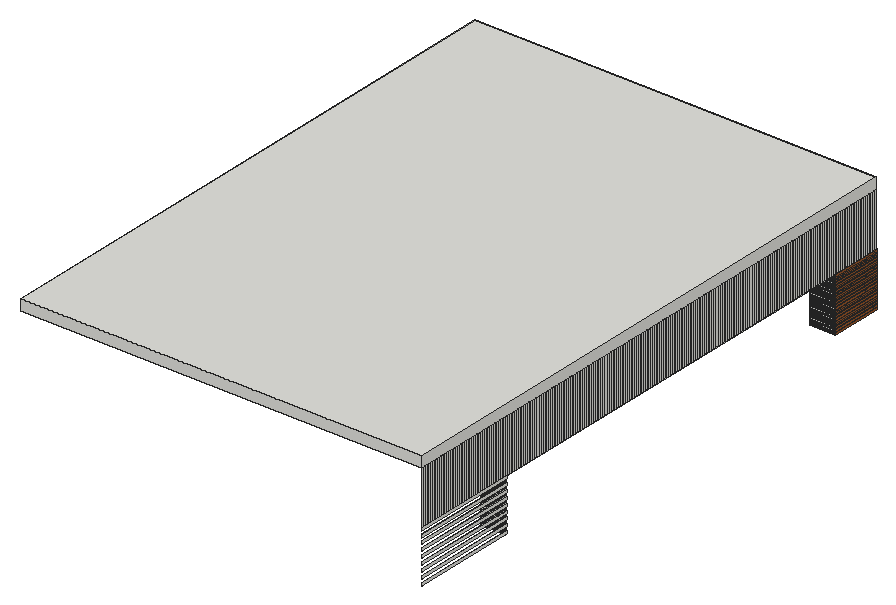
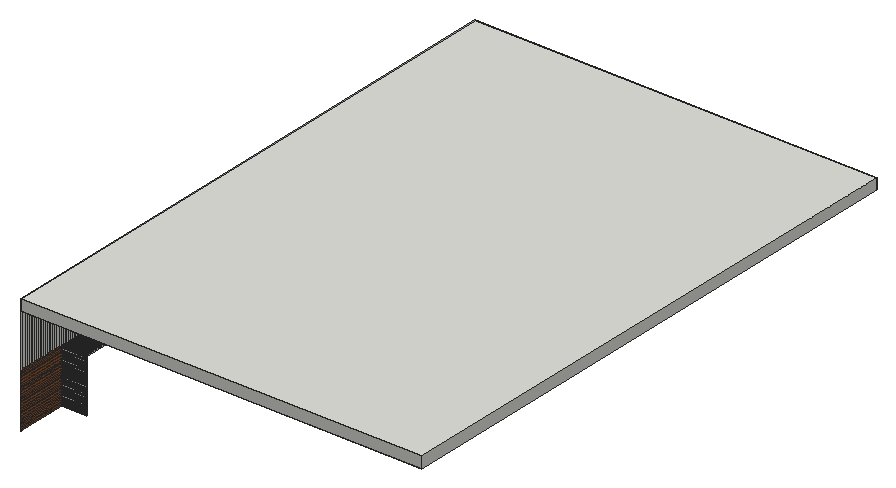
# SketchUp Ruby script. Lengths in inches.
U = 1.inch
M = Sketchup.active_model
def pt(a) = Geom::Point3d.new(a.map { |v| v * U })
def face(e, loops, mat)
  f = e.add_face(loops[0].map { |a| pt(a) })
  loops[1..].each { |l| e.add_face(l.map { |a| pt(a) }).erase! }
  f.material = f.back_material = mat if mat
  f
end
# faces: each face lists its corners as indices into pts; further lists are holes
def faces(e, pts, list, mat = nil) = list.each { |f| face(e, (f[0].is_a?(Array) ? f : [f]).map { |l| l.map { |i| pts[i] } }, mat) }
# xy, xz, yz: faces in a plane at the given z, y or x. An outline is a flat list of corners, or four numbers for a rectangle; further outlines are holes
def ring(l) = l.size == 4 ? [[l[0], l[1]], [l[2], l[1]], [l[2], l[3]], [l[0], l[3]]] : l.each_slice(2).to_a
def flat(e, list, mat, &to3) = list.each { |f| face(e, (f[0].is_a?(Array) ? f : [f]).map { |l| ring(l).map { |u, v| to3.(u, v) } }, mat) }
def xy(e, z, list, mat = nil) = flat(e, list, mat) { |x, y| [x, y, z] }
def xz(e, y, list, mat = nil) = flat(e, list, mat) { |x, z| [x, y, z] }
def yz(e, x, list, mat = nil) = flat(e, list, mat) { |y, z| [x, y, z] }
def lines(e, pts, list) = list.each { |a, b| e.add_line(pt(pts[a]), pt(pts[b])) }
# prism: a flat outline (further loops are holes) pulled along v
def prism(e, loops, v, mat = nil)
  f = face(e, loops, mat); d = Geom::Vector3d.new(v.map { |x| x * U })
  f.pushpull(f.normal.samedirection?(d) ? d.length : -d.length)
end
def box(e, o, s, mat = nil) = prism(e, [[o, [o[0] + s[0], o[1], o[2]], [o[0] + s[0], o[1] + s[1], o[2]], [o[0], o[1] + s[1], o[2]]]], [0, 0, s[2]], mat)
def at(x, y, z, deg = 0) = Geom::Transformation.translation(pt([x, y, z])) * Geom::Transformation.rotation(ORIGIN, Z_AXIS, deg.degrees)
def axes(o, x, y, z) = Geom::Transformation.new([*x, 0, *y, 0, *z, 0, *pt(o).to_a, 1])
def part(name) = M.definitions.add(name)
# library, detail: a bought-in or finely detailed component or shape, given as its bounding box
def library(name, o, s) = part(name).tap { |d| box(d.entities, o, s) }
def detail(e, o, s) = box(e.add_group.entities, o, s)
def put(e, d, t, mat = nil) = e.add_instance(d, t).tap { |i| i.material = mat if mat }
def group(e, t, mat = nil) = e.add_group.tap { |g| g.transformation = t; g.material = mat if mat }.entities
root = M.entities
M.materials.add("Emissive").color = [255, 185, 108]
M.materials.add("[Wood Cherry Original]").color = [152, 86, 42]
c1 = part("Group\#16")
box(c1.entities,[0,0,0],[0.125,18.33,0.46])
c2 = part("Group\#10")
box(c2.entities,[0,0,0],[9,0.1875,0.36])
c3 = part("Group\#8")
box(c3.entities,[0,0,0],[0.25,37.84,0.98])
c4 = part("Group\#9")
box(c4.entities,[0,0,0],[0.125,0.46,19.02])
c5 = library("Group\#21",[-0.5,-0.5,0],[72.18,132.18,1.5625])
put(root,c1,at(144,185.67,81.44),"[Wood Cherry Original]")
put(root,c2,at(135,185.48,81.53))
put(root,c2,at(135,37.84,81.86))
put(root,c1,at(144,185.67,81.95),"[Wood Cherry Original]")
put(root,c2,at(135,185.48,82.03))
put(root,c3,at(144,0,82.22))
put(root,c1,at(144,185.67,82.45),"[Wood Cherry Original]")
put(root,c2,at(135,37.84,82.53))
put(root,c2,at(135,185.48,82.53))
put(root,c1,at(144,185.67,82.95),"[Wood Cherry Original]")
put(root,c2,at(135,185.48,83.04))
put(root,c2,at(135,37.84,83.2))
put(root,c1,at(144,185.67,83.46),"[Wood Cherry Original]")
put(root,c2,at(135,185.48,83.54))
put(root,c2,at(135,37.84,83.875))
put(root,c1,at(144,185.67,83.96),"[Wood Cherry Original]")
put(root,c2,at(135,185.48,84.04))
put(root,c3,at(144,0,84.44))
put(root,c1,at(144,185.67,84.46),"[Wood Cherry Original]")
put(root,c2,at(135,37.84,84.54))
put(root,c2,at(135,185.48,84.54))
put(root,c1,at(144,185.67,84.96),"[Wood Cherry Original]")
put(root,c2,at(135,185.48,85.05))
put(root,c2,at(135,37.84,85.22))
put(root,c1,at(144,185.67,85.47),"[Wood Cherry Original]")
put(root,c2,at(135,185.48,85.55))
put(root,c2,at(135,37.84,85.89))
put(root,c1,at(144,185.67,85.97),"[Wood Cherry Original]")
put(root,c2,at(135,185.48,86.05))
put(root,c1,at(144,185.67,86.47),"[Wood Cherry Original]")
put(root,c2,at(135,37.84,86.56))
put(root,c2,at(135,185.48,86.56))
put(root,c3,at(144,0,86.67))
put(root,c1,at(144,185.67,86.97),"[Wood Cherry Original]")
put(root,c2,at(135,185.48,87.0625))
put(root,c2,at(135,37.84,87.23))
put(root,c1,at(144,185.67,87.48),"[Wood Cherry Original]")
put(root,c2,at(135,185.48,87.5625))
put(root,c2,at(135,37.84,87.9))
put(root,c1,at(144,185.67,87.98),"[Wood Cherry Original]")
put(root,c2,at(135,185.48,88.07))
g1 = group(root,at(144,185.67,88.48),"[Wood Cherry Original]")
box(g1,[0,0,0],[0.125,18.33,0.46])
put(root,c2,at(135,37.84,88.57))
put(root,c2,at(135,185.48,88.57))
put(root,c3,at(144,0,88.89))
put(root,c1,at(144,185.67,88.99),"[Wood Cherry Original]")
put(root,c2,at(135,185.48,89.07))
put(root,c2,at(135,37.84,89.24))
put(root,c1,at(144,185.67,89.49),"[Wood Cherry Original]")
put(root,c2,at(135,185.48,89.58))
put(root,c2,at(135,37.84,89.91))
put(root,c1,at(144,185.67,89.99),"[Wood Cherry Original]")
put(root,c2,at(135,185.48,90.08))
put(root,c1,at(144,185.67,90.49),"[Wood Cherry Original]")
put(root,c2,at(135,37.84,90.58))
put(root,c2,at(135,185.48,90.58))
put(root,c1,at(144,185.67,91),"[Wood Cherry Original]")
put(root,c2,at(135,185.48,91.09))
put(root,c3,at(144,0,91.11))
put(root,c2,at(135,37.84,91.25))
put(root,c1,at(144,185.67,91.5),"[Wood Cherry Original]")
put(root,c2,at(135,185.48,91.59))
put(root,c2,at(135,37.84,91.93))
put(root,c1,at(144,185.67,92),"[Wood Cherry Original]")
put(root,c2,at(135,185.48,92.09))
put(root,c1,at(144,185.67,92.51),"[Wood Cherry Original]")
put(root,c2,at(135,37.84,92.6))
put(root,c2,at(135,185.48,92.6))
g2 = group(root,at(144,185.67,93.01),"[Wood Cherry Original]")
box(g2,[0,0,0],[0.125,18.33,0.46])
put(root,c2,at(135,185.48,93.1))
put(root,c2,at(135,37.84,93.27))
put(root,c3,at(144,0,93.33))
put(root,c1,at(144,185.67,93.51),"[Wood Cherry Original]")
put(root,c2,at(135,185.48,93.6))
put(root,c2,at(135,37.84,93.9375))
put(root,c1,at(144,185.67,94.01),"[Wood Cherry Original]")
put(root,c2,at(135,185.48,94.11))
put(root,c1,at(144,185.67,94.52),"[Wood Cherry Original]")
put(root,c2,at(135,37.84,94.61))
put(root,c2,at(135,185.48,94.61))
put(root,c1,at(144,185.67,95.02),"[Wood Cherry Original]")
put(root,c2,at(135,185.48,95.11))
put(root,c2,at(135,37.84,95.28))
put(root,c1,at(144,185.67,95.52),"[Wood Cherry Original]")
put(root,c3,at(144,0,95.56))
put(root,c2,at(135,185.48,95.62))
put(root,c2,at(135,37.84,95.95))
put(root,c1,at(144,185.67,96.02),"[Wood Cherry Original]")
put(root,c2,at(135,185.48,96.12))
put(root,c1,at(144,185.67,96.53),"[Wood Cherry Original]")
put(root,c2,at(135,37.84,96.62))
put(root,c2,at(135,185.48,96.62))
put(root,c1,at(144,185.67,97.03),"[Wood Cherry Original]")
put(root,c2,at(135,185.48,97.125))
put(root,c2,at(135,37.84,97.29))
put(root,c1,at(144,185.67,97.53),"[Wood Cherry Original]")
put(root,c2,at(135,185.48,97.63))
put(root,c3,at(144,0,97.78))
put(root,c2,at(135,37.84,97.96))
put(root,c1,at(144,185.67,98.04),"[Wood Cherry Original]")
put(root,c2,at(135,185.48,98.13))
put(root,c1,at(144,185.67,98.54),"[Wood Cherry Original]")
put(root,c2,at(135,37.84,98.64))
put(root,c2,at(135,185.48,98.64))
put(root,c1,at(144,185.67,99.04),"[Wood Cherry Original]")
put(root,c2,at(135,185.48,99.14))
put(root,c2,at(135,37.84,99.31))
put(root,c1,at(144,185.67,99.54),"[Wood Cherry Original]")
put(root,c2,at(135,185.48,99.64))
put(root,c2,at(135,37.84,99.98))
put(root,c3,at(144,0,100))
put(root,c1,at(144,185.67,100.05),"[Wood Cherry Original]")
put(root,c2,at(135,185.48,100.15))
put(root,c1,at(144,185.67,100.55),"[Wood Cherry Original]")
put(root,c2,at(135,185.11,100.62))
put(root,c2,at(135,184.38,100.62))
put(root,c2,at(135,183.64,100.62))
put(root,c2,at(135,182.91,100.62))
put(root,c2,at(135,182.17,100.62))
put(root,c2,at(135,181.4375,100.62))
put(root,c2,at(135,180.7,100.62))
put(root,c2,at(135,179.97,100.62))
put(root,c2,at(135,179.23,100.62))
put(root,c2,at(135,178.5,100.62))
put(root,c2,at(135,177.76,100.62))
put(root,c2,at(135,177.03,100.62))
put(root,c2,at(135,176.29,100.62))
put(root,c2,at(135,175.56,100.62))
put(root,c2,at(135,174.82,100.62))
put(root,c2,at(135,174.09,100.62))
put(root,c2,at(135,173.35,100.62))
put(root,c2,at(135,172.62,100.62))
put(root,c2,at(135,171.88,100.62))
put(root,c2,at(135,171.15,100.62))
put(root,c2,at(135,170.41,100.62))
put(root,c2,at(135,169.67,100.62))
put(root,c2,at(135,168.94,100.62))
put(root,c2,at(135,168.2,100.62))
put(root,c2,at(135,167.47,100.62))
put(root,c2,at(135,166.73,100.62))
put(root,c2,at(135,166,100.62))
put(root,c2,at(135,165.26,100.625))
put(root,c2,at(135,164.53,100.625))
put(root,c2,at(135,163.79,100.625))
put(root,c2,at(135,163.06,100.625))
put(root,c2,at(135,162.32,100.625))
put(root,c2,at(135,161.59,100.625))
put(root,c2,at(135,160.85,100.625))
put(root,c2,at(135,160.12,100.625))
put(root,c2,at(135,159.38,100.625))
put(root,c2,at(135,158.65,100.625))
put(root,c2,at(135,157.91,100.625))
put(root,c2,at(135,157.18,100.625))
put(root,c2,at(135,156.44,100.625))
put(root,c2,at(135,155.71,100.625))
put(root,c2,at(135,154.97,100.625))
put(root,c2,at(135,154.24,100.625))
put(root,c2,at(135,153.5,100.625))
put(root,c2,at(135,152.77,100.625))
put(root,c2,at(135,152.03,100.625))
put(root,c2,at(135,151.3,100.625))
put(root,c2,at(135,150.5625,100.625))
put(root,c2,at(135,149.83,100.625))
put(root,c2,at(135,149.09,100.625))
put(root,c2,at(135,148.36,100.625))
put(root,c2,at(135,147.62,100.625))
put(root,c2,at(135,146.89,100.625))
put(root,c2,at(135,146.15,100.625))
put(root,c2,at(135,145.41,100.63))
put(root,c2,at(135,144.68,100.63))
put(root,c2,at(135,143.94,100.63))
put(root,c2,at(135,143.21,100.63))
put(root,c2,at(135,142.47,100.63))
put(root,c2,at(135,141.74,100.63))
put(root,c2,at(135,141,100.63))
put(root,c2,at(135,140.27,100.63))
put(root,c2,at(135,139.53,100.63))
put(root,c2,at(135,138.8,100.63))
put(root,c2,at(135,138.0625,100.63))
put(root,c2,at(135,137.33,100.63))
put(root,c2,at(135,136.59,100.63))
put(root,c2,at(135,135.86,100.63))
put(root,c2,at(135,135.12,100.63))
put(root,c2,at(135,134.39,100.63))
put(root,c2,at(135,133.65,100.63))
put(root,c2,at(135,132.92,100.63))
put(root,c2,at(135,132.18,100.63))
put(root,c2,at(135,131.45,100.63))
put(root,c2,at(135,130.71,100.63))
put(root,c2,at(135,129.98,100.63))
put(root,c2,at(135,129.24,100.63))
put(root,c2,at(135,128.51,100.63))
put(root,c2,at(135,127.77,100.63))
put(root,c2,at(135,127.04,100.63))
put(root,c2,at(135,126.3,100.63))
put(root,c2,at(135,125.57,100.63))
put(root,c2,at(135,124.83,100.63))
put(root,c2,at(135,124.1,100.63))
put(root,c2,at(135,123.36,100.63))
put(root,c2,at(135,122.625,100.63))
put(root,c2,at(135,121.89,100.63))
put(root,c2,at(135,121.15,100.63))
put(root,c2,at(135,120.42,100.63))
put(root,c2,at(135,119.68,100.63))
put(root,c2,at(135,118.95,100.63))
put(root,c2,at(135,118.21,100.63))
put(root,c2,at(135,117.48,100.63))
put(root,c2,at(135,116.74,100.63))
put(root,c2,at(135,116.01,100.63))
put(root,c2,at(135,115.27,100.63))
put(root,c2,at(135,114.54,100.63))
put(root,c2,at(135,113.8,100.63))
put(root,c2,at(135,113.07,100.63))
put(root,c2,at(135,112.33,100.63))
put(root,c2,at(135,111.6,100.63))
put(root,c2,at(135,110.86,100.63))
put(root,c2,at(135,110.13,100.63))
put(root,c2,at(135,109.39,100.63))
put(root,c2,at(135,108.66,100.63))
put(root,c2,at(135,107.92,100.63))
put(root,c2,at(135,107.1875,100.63))
put(root,c2,at(135,106.45,100.63))
put(root,c2,at(135,105.72,100.64))
put(root,c2,at(135,104.98,100.64))
put(root,c2,at(135,104.25,100.64))
put(root,c2,at(135,103.51,100.64))
put(root,c2,at(135,102.78,100.64))
put(root,c2,at(135,102.04,100.64))
put(root,c2,at(135,101.31,100.64))
put(root,c2,at(135,100.57,100.64))
put(root,c2,at(135,99.84,100.64))
put(root,c2,at(135,99.1,100.64))
put(root,c2,at(135,98.37,100.64))
put(root,c2,at(135,97.63,100.64))
put(root,c2,at(135,96.89,100.64))
put(root,c2,at(135,96.16,100.64))
put(root,c2,at(135,95.42,100.64))
put(root,c2,at(135,94.6875,100.64))
put(root,c2,at(135,93.95,100.64))
put(root,c2,at(135,93.22,100.64))
put(root,c2,at(135,92.48,100.64))
put(root,c2,at(135,91.75,100.64))
put(root,c2,at(135,91.01,100.64))
put(root,c2,at(135,90.28,100.64))
put(root,c2,at(135,89.54,100.64))
put(root,c2,at(135,88.81,100.64))
put(root,c2,at(135,88.07,100.64))
put(root,c2,at(135,87.34,100.64))
put(root,c2,at(135,86.6,100.64))
put(root,c2,at(135,85.87,100.64))
put(root,c2,at(135,85.13,100.64))
put(root,c2,at(135,84.4,100.64))
put(root,c2,at(135,83.66,100.64))
put(root,c2,at(135,82.93,100.64))
put(root,c2,at(135,82.19,100.64))
put(root,c2,at(135,81.46,100.64))
put(root,c2,at(135,80.72,100.64))
put(root,c2,at(135,79.99,100.64))
put(root,c2,at(135,79.25,100.64))
put(root,c2,at(135,78.52,100.64))
put(root,c2,at(135,77.78,100.64))
put(root,c2,at(135,77.05,100.64))
put(root,c2,at(135,76.3125,100.64))
put(root,c2,at(135,75.58,100.64))
put(root,c2,at(135,74.84,100.64))
put(root,c2,at(135,74.11,100.64))
put(root,c2,at(135,73.37,100.64))
put(root,c2,at(135,72.63,100.64))
put(root,c2,at(135,71.9,100.64))
put(root,c2,at(135,71.16,100.64))
put(root,c2,at(135,70.43,100.64))
put(root,c2,at(135,69.69,100.64))
put(root,c2,at(135,68.96,100.64))
put(root,c2,at(135,68.22,100.64))
put(root,c2,at(135,67.49,100.64))
put(root,c2,at(135,66.75,100.64))
put(root,c2,at(135,66.02,100.64))
put(root,c2,at(135,65.28,100.64))
put(root,c2,at(135,64.55,100.64))
put(root,c2,at(135,63.8125,100.64))
put(root,c2,at(135,63.08,100.64))
put(root,c2,at(135,62.34,100.64))
put(root,c2,at(135,61.61,100.64))
put(root,c2,at(135,60.87,100.64))
put(root,c2,at(135,60.14,100.64))
put(root,c2,at(135,59.4,100.64))
put(root,c2,at(135,58.67,100.64))
put(root,c2,at(135,57.93,100.64))
put(root,c2,at(135,57.2,100.64))
put(root,c2,at(135,56.46,100.64))
put(root,c2,at(135,55.73,100.65))
put(root,c2,at(135,54.99,100.65))
put(root,c2,at(135,54.26,100.65))
put(root,c2,at(135,53.52,100.65))
put(root,c2,at(135,52.79,100.65))
put(root,c2,at(135,52.05,100.65))
put(root,c2,at(135,51.32,100.65))
put(root,c2,at(135,50.58,100.65))
put(root,c2,at(135,49.85,100.65))
put(root,c2,at(135,49.11,100.65))
put(root,c2,at(135,48.375,100.65))
put(root,c2,at(135,47.64,100.65))
put(root,c2,at(135,46.9,100.65))
put(root,c2,at(135,46.17,100.65))
put(root,c2,at(135,45.43,100.65))
put(root,c2,at(135,44.7,100.65))
put(root,c2,at(135,43.96,100.65))
put(root,c2,at(135,43.23,100.65))
put(root,c2,at(135,42.49,100.65))
put(root,c2,at(135,41.76,100.65))
put(root,c2,at(135,41.02,100.65))
put(root,c2,at(135,40.29,100.65))
put(root,c2,at(135,39.55,100.65))
put(root,c2,at(135,38.82,100.65))
put(root,c2,at(135,37.84,100.65))
put(root,c2,at(135,185.48,100.65))
put(root,c2,at(135,38.08,100.65))
put(root,c4,at(144,0,100.98))
put(root,c4,at(144,1.02,100.98))
put(root,c4,at(144,2.03,100.98))
put(root,c4,at(144,3.05,100.98))
put(root,c4,at(144,4.07,100.98))
put(root,c4,at(144,5.08,100.98))
put(root,c4,at(144,6.1,100.98))
put(root,c4,at(144,7.12,100.98))
put(root,c4,at(144,8.14,100.98))
put(root,c4,at(144,9.15,100.98))
put(root,c4,at(144,10.17,100.98))
put(root,c4,at(144,11.1875,100.98))
put(root,c4,at(144,12.2,100.98))
put(root,c4,at(144,13.22,100.98))
put(root,c4,at(144,14.24,100.98))
put(root,c4,at(144,15.25,100.98))
put(root,c4,at(144,16.27,100.98))
put(root,c4,at(144,17.29,100.98))
put(root,c4,at(144,18.3,100.98))
put(root,c4,at(144,19.32,100.98))
put(root,c4,at(144,20.34,100.98))
put(root,c4,at(144,21.35,100.98))
put(root,c4,at(144,22.37,100.98))
put(root,c4,at(144,23.39,100.98))
put(root,c4,at(144,24.4,100.98))
put(root,c4,at(144,25.42,100.98))
put(root,c4,at(144,26.4375,100.98))
put(root,c4,at(144,27.46,100.98))
put(root,c4,at(144,28.47,100.98))
put(root,c4,at(144,29.49,100.98))
put(root,c4,at(144,30.51,100.98))
put(root,c4,at(144,31.52,100.98))
put(root,c4,at(144,32.54,100.98))
put(root,c4,at(144,33.56,100.98))
put(root,c4,at(144,34.57,100.98))
put(root,c4,at(144,35.59,100.98))
put(root,c4,at(144,36.61,100.98))
put(root,c4,at(144,37.625,100.98))
put(root,c4,at(144,38.64,100.98))
put(root,c4,at(144,39.66,100.98))
put(root,c4,at(144,40.67,100.98))
put(root,c4,at(144,41.69,100.98))
put(root,c4,at(144,42.71,100.98))
put(root,c4,at(144,43.73,100.98))
put(root,c4,at(144,44.74,100.98))
put(root,c4,at(144,45.76,100.98))
put(root,c4,at(144,46.78,100.98))
put(root,c4,at(144,47.79,100.98))
put(root,c4,at(144,48.81,100.98))
put(root,c4,at(144,49.83,100.98))
put(root,c4,at(144,50.84,100.98))
put(root,c4,at(144,51.86,100.98))
put(root,c4,at(144,52.88,100.98))
put(root,c4,at(144,53.89,100.98))
put(root,c4,at(144,54.91,100.98))
put(root,c4,at(144,55.93,100.98))
put(root,c4,at(144,56.94,100.98))
put(root,c4,at(144,57.96,100.98))
put(root,c4,at(144,58.98,100.98))
put(root,c4,at(144,60,100.98))
put(root,c4,at(144,61.01,100.98))
put(root,c4,at(144,62.03,100.98))
put(root,c4,at(144,63.05,100.98))
put(root,c4,at(144,64.0625,100.98))
put(root,c4,at(144,65.08,100.98))
put(root,c4,at(144,66.1,100.98))
put(root,c4,at(144,67.11,100.98))
put(root,c4,at(144,68.13,100.98))
put(root,c4,at(144,69.15,100.98))
put(root,c4,at(144,70.16,100.98))
put(root,c4,at(144,71.18,100.98))
put(root,c4,at(144,72.2,100.98))
put(root,c4,at(144,73.21,100.98))
put(root,c4,at(144,74.23,100.98))
put(root,c4,at(144,75.25,100.98))
put(root,c4,at(144,76.27,100.98))
put(root,c4,at(144,77.28,100.98))
put(root,c4,at(144,78.3,100.98))
put(root,c4,at(144,79.32,100.98))
put(root,c4,at(144,80.33,100.98))
put(root,c4,at(144,81.35,100.98))
put(root,c4,at(144,82.37,100.98))
put(root,c4,at(144,83.38,100.98))
put(root,c4,at(144,84.4,100.98))
put(root,c4,at(144,85.42,100.98))
put(root,c4,at(144,86.43,100.98))
put(root,c4,at(144,87.45,100.98))
put(root,c4,at(144,88.47,100.98))
put(root,c4,at(144,89.48,100.98))
put(root,c4,at(144,90.5,100.98))
put(root,c4,at(144,91.52,100.98))
put(root,c4,at(144,92.54,100.98))
put(root,c4,at(144,93.55,100.98))
put(root,c4,at(144,94.57,100.98))
put(root,c4,at(144,95.59,100.98))
put(root,c4,at(144,96.6,100.98))
put(root,c4,at(144,97.62,100.98))
put(root,c4,at(144,98.64,100.98))
put(root,c4,at(144,99.65,100.98))
put(root,c4,at(144,100.67,100.98))
put(root,c4,at(144,101.6875,100.98))
put(root,c4,at(144,102.7,100.98))
put(root,c4,at(144,103.72,100.98))
put(root,c4,at(144,104.74,100.98))
put(root,c4,at(144,105.75,100.98))
put(root,c4,at(144,106.77,100.98))
put(root,c4,at(144,107.79,100.98))
put(root,c4,at(144,108.81,100.98))
put(root,c4,at(144,109.82,100.98))
put(root,c4,at(144,110.84,100.98))
put(root,c4,at(144,111.86,100.98))
put(root,c4,at(144,112.875,100.98))
put(root,c4,at(144,113.89,100.98))
put(root,c4,at(144,114.91,100.98))
put(root,c4,at(144,115.92,100.98))
put(root,c4,at(144,116.94,100.98))
put(root,c4,at(144,117.96,100.98))
put(root,c4,at(144,118.97,100.98))
put(root,c4,at(144,119.99,100.98))
put(root,c4,at(144,121.01,100.98))
put(root,c4,at(144,122.02,100.98))
put(root,c4,at(144,123.04,100.98))
put(root,c4,at(144,124.06,100.98))
put(root,c4,at(144,125.08,100.98))
put(root,c4,at(144,126.09,100.98))
put(root,c4,at(144,127.11,100.98))
put(root,c4,at(144,128.125,100.98))
put(root,c4,at(144,129.14,100.98))
put(root,c4,at(144,130.16,100.98))
put(root,c4,at(144,131.18,100.98))
put(root,c4,at(144,132.19,100.98))
put(root,c4,at(144,133.21,100.98))
put(root,c4,at(144,134.23,100.98))
put(root,c4,at(144,135.24,100.98))
put(root,c4,at(144,136.26,100.98))
put(root,c4,at(144,137.28,100.98))
put(root,c4,at(144,138.29,100.98))
put(root,c4,at(144,139.3125,100.98))
put(root,c4,at(144,140.33,100.98))
put(root,c4,at(144,141.35,100.98))
put(root,c4,at(144,142.36,100.98))
put(root,c4,at(144,143.38,100.98))
put(root,c4,at(144,144.4,100.98))
put(root,c4,at(144,145.41,100.98))
put(root,c4,at(144,146.43,100.98))
put(root,c4,at(144,147.45,100.98))
put(root,c4,at(144,148.46,100.98))
put(root,c4,at(144,149.48,100.98))
put(root,c4,at(144,150.5,100.98))
put(root,c4,at(144,151.51,100.98))
put(root,c4,at(144,152.53,100.98))
put(root,c4,at(144,153.55,100.98))
put(root,c4,at(144,154.56,100.98))
put(root,c4,at(144,155.58,100.98))
put(root,c4,at(144,156.6,100.98))
put(root,c4,at(144,157.62,100.98))
put(root,c4,at(144,158.63,100.98))
put(root,c4,at(144,159.65,100.98))
put(root,c4,at(144,160.67,100.98))
put(root,c4,at(144,161.68,100.98))
put(root,c4,at(144,162.7,100.98))
put(root,c4,at(144,163.72,100.98))
put(root,c4,at(144,164.73,100.98))
put(root,c4,at(144,165.75,100.98))
put(root,c4,at(144,166.77,100.98))
put(root,c4,at(144,167.78,100.98))
put(root,c4,at(144,168.8,100.98))
put(root,c4,at(144,169.82,100.98))
put(root,c4,at(144,170.83,100.98))
put(root,c4,at(144,171.85,100.98))
put(root,c4,at(144,172.87,100.98))
put(root,c4,at(144,173.89,100.98))
put(root,c4,at(144,174.9,100.98))
put(root,c4,at(144,175.92,100.98))
put(root,c4,at(144,176.9375,100.98))
put(root,c4,at(144,177.95,100.98))
put(root,c4,at(144,178.97,100.98))
put(root,c4,at(144,179.99,100.98))
put(root,c4,at(144,181,100.98))
put(root,c4,at(144,182.02,100.98))
put(root,c4,at(144,183.04,100.98))
put(root,c4,at(144,184.05,100.98))
put(root,c4,at(144,185.07,100.98))
put(root,c4,at(144,186.09,100.98))
put(root,c4,at(144,187.1,100.98))
put(root,c4,at(144,188.12,100.98))
put(root,c4,at(144,189.14,100.98))
put(root,c4,at(144,190.16,100.98))
put(root,c4,at(144,191.17,100.98))
put(root,c4,at(144,192.1875,100.98))
put(root,c4,at(144,193.21,100.98))
put(root,c4,at(144,194.22,100.98))
put(root,c4,at(144,195.24,100.98))
put(root,c4,at(144,196.26,100.98))
put(root,c4,at(144,197.27,100.98))
put(root,c4,at(144,198.29,100.98))
put(root,c4,at(144,199.31,100.98))
put(root,c4,at(144,200.32,100.98))
put(root,c4,at(144,201.34,100.98))
put(root,c4,at(144,202.36,100.98))
put(root,c4,at(144,203.375,100.98))
g3 = group(root,at(0,0,120))
xy(g3,0,[[[0,0,144,204],[38.91,38.91,105.09,165.09],[53.19,8.6,57.5,15.58],[87.29,8.6,91.61,15.58],[121.4,8.6,125.71,15.58],[121.4,65.79,125.71,72.77],[121.4,122.98,125.71,129.95],[121.4,180.16,125.71,187.14],[87.07,180.16,91.38,187.14],[52.73,180.16,57.04,187.14],[18.4,180.16,22.71,187.14],[18.63,122.98,22.94,129.95],[18.86,65.79,23.17,72.77],[18.86,8.98,23.17,15.95]]])
xy(g3,1.1875,[[18.86,8.98,23.17,15.95],[18.86,65.79,23.17,72.77]],"Emissive")
xy(g3,1.5625,[[36.41,36.41,38.91,165.09],[38.91,36.41,105.09,38.91],[105.09,36.41,107.59,165.09],[36.41,165.09,107.59,167.59]])
xy(g3,1.5625,[[53.19,8.6,57.5,15.58],[87.29,8.6,91.61,15.58],[121.4,8.6,125.71,15.58],[121.4,65.79,125.71,72.77],[18.63,122.98,22.94,129.95],
  [121.4,122.98,125.71,129.95],[18.4,180.16,22.71,187.14],[52.73,180.16,57.04,187.14],[87.07,180.16,91.38,187.14],[121.4,180.16,125.71,187.14]],"Emissive")
xy(g3,3.125,[[36.41,36.41,107.59,167.59]])
xy(g3,4,[[0,0,144,204]])
xz(g3,0,[[0,0,144,4]])
xz(g3,8.6,[[53.19,0,57.5,1.5625],[87.29,0,91.61,1.5625],[121.4,0,125.71,1.5625]],"Emissive")
xz(g3,8.98,[[18.86,0,23.17,1.1875]],"Emissive")
xz(g3,15.58,[[53.19,0,57.5,1.5625],[87.29,0,91.61,1.5625],[121.4,0,125.71,1.5625]],"Emissive")
xz(g3,15.95,[[18.86,0,23.17,1.1875]],"Emissive")
xz(g3,38.91,[[38.91,0,105.09,1.5625]])
xz(g3,65.79,[[18.86,0,23.17,1.1875],[121.4,0,125.71,1.5625]],"Emissive")
xz(g3,72.77,[[18.86,0,23.17,1.1875],[121.4,0,125.71,1.5625]],"Emissive")
xz(g3,122.98,[[18.63,0,22.94,1.5625],[121.4,0,125.71,1.5625]],"Emissive")
xz(g3,129.95,[[18.63,0,22.94,1.5625],[121.4,0,125.71,1.5625]],"Emissive")
xz(g3,165.09,[[38.91,0,105.09,1.5625]])
xz(g3,180.16,[[18.4,0,22.71,1.5625],[52.73,0,57.04,1.5625],[87.07,0,91.38,1.5625],[121.4,0,125.71,1.5625]],"Emissive")
xz(g3,187.14,[[18.4,0,22.71,1.5625],[52.73,0,57.04,1.5625],[87.07,0,91.38,1.5625],[121.4,0,125.71,1.5625]],"Emissive")
xz(g3,204,[[0,0,144,4]])
yz(g3,0,[[0,0,204,4]])
yz(g3,18.4,[[180.16,0,187.14,1.5625]],"Emissive")
yz(g3,18.63,[[122.98,0,129.95,1.5625]],"Emissive")
yz(g3,18.86,[[8.98,0,15.95,1.1875],[65.79,0,72.77,1.1875]],"Emissive")
yz(g3,22.71,[[180.16,0,187.14,1.5625]],"Emissive")
yz(g3,22.94,[[122.98,0,129.95,1.5625]],"Emissive")
yz(g3,23.17,[[8.98,0,15.95,1.1875],[65.79,0,72.77,1.1875]],"Emissive")
yz(g3,38.91,[[38.91,0,165.09,1.5625]])
yz(g3,52.73,[[180.16,0,187.14,1.5625]],"Emissive")
yz(g3,53.19,[[8.6,0,15.58,1.5625]],"Emissive")
yz(g3,57.04,[[180.16,0,187.14,1.5625]],"Emissive")
yz(g3,57.5,[[8.6,0,15.58,1.5625]],"Emissive")
yz(g3,87.07,[[180.16,0,187.14,1.5625]],"Emissive")
yz(g3,87.29,[[8.6,0,15.58,1.5625]],"Emissive")
yz(g3,91.38,[[180.16,0,187.14,1.5625]],"Emissive")
yz(g3,91.61,[[8.6,0,15.58,1.5625]],"Emissive")
yz(g3,105.09,[[38.91,0,165.09,1.5625]])
yz(g3,121.4,[[8.6,0,15.58,1.5625],[65.79,0,72.77,1.5625],[122.98,0,129.95,1.5625],[180.16,0,187.14,1.5625]],"Emissive")
yz(g3,125.71,[[8.6,0,15.58,1.5625],[65.79,0,72.77,1.5625],[122.98,0,129.95,1.5625],[180.16,0,187.14,1.5625]],"Emissive")
yz(g3,144,[[0,0,204,4]])
put(g3,c5,at(36.41,36.41,1.5625))
